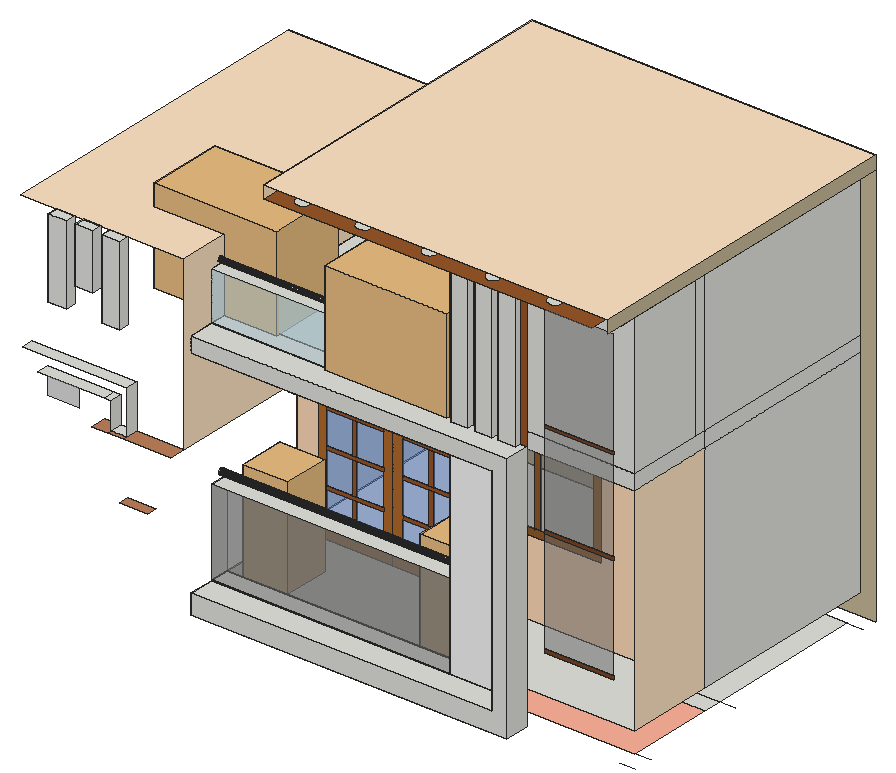
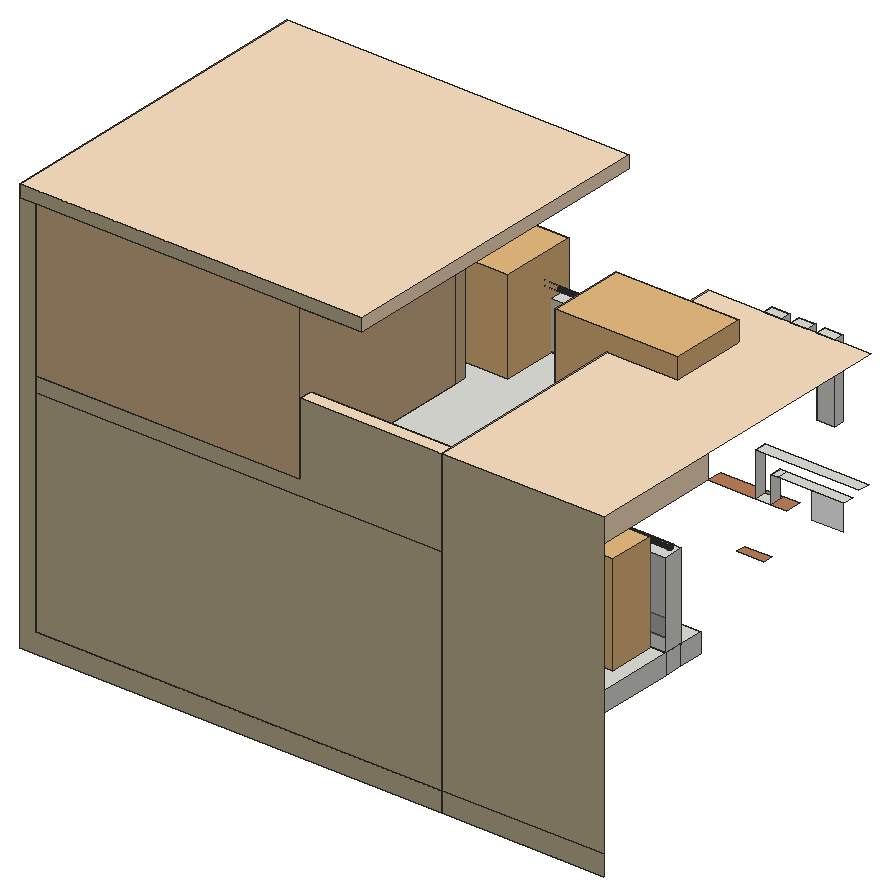
# SketchUp Ruby script. Lengths in inches.
U = 1.inch
M = Sketchup.active_model
def pt(a) = Geom::Point3d.new(a.map { |v| v * U })
def face(e, loops, mat)
  f = e.add_face(loops[0].map { |a| pt(a) })
  loops[1..].each { |l| e.add_face(l.map { |a| pt(a) }).erase! }
  f.material = f.back_material = mat if mat
  f
end
# faces: each face lists its corners as indices into pts; further lists are holes
def faces(e, pts, list, mat = nil) = list.each { |f| face(e, (f[0].is_a?(Array) ? f : [f]).map { |l| l.map { |i| pts[i] } }, mat) }
# xy, xz, yz: faces in a plane at the given z, y or x. An outline is a flat list of corners, or four numbers for a rectangle; further outlines are holes
def ring(l) = l.size == 4 ? [[l[0], l[1]], [l[2], l[1]], [l[2], l[3]], [l[0], l[3]]] : l.each_slice(2).to_a
def flat(e, list, mat, &to3) = list.each { |f| face(e, (f[0].is_a?(Array) ? f : [f]).map { |l| ring(l).map { |u, v| to3.(u, v) } }, mat) }
def xy(e, z, list, mat = nil) = flat(e, list, mat) { |x, y| [x, y, z] }
def xz(e, y, list, mat = nil) = flat(e, list, mat) { |x, z| [x, y, z] }
def yz(e, x, list, mat = nil) = flat(e, list, mat) { |y, z| [x, y, z] }
def lines(e, pts, list) = list.each { |a, b| e.add_line(pt(pts[a]), pt(pts[b])) }
# prism: a flat outline (further loops are holes) pulled along v
def prism(e, loops, v, mat = nil)
  f = face(e, loops, mat); d = Geom::Vector3d.new(v.map { |x| x * U })
  f.pushpull(f.normal.samedirection?(d) ? d.length : -d.length)
end
def box(e, o, s, mat = nil) = prism(e, [[o, [o[0] + s[0], o[1], o[2]], [o[0] + s[0], o[1] + s[1], o[2]], [o[0], o[1] + s[1], o[2]]]], [0, 0, s[2]], mat)
def at(x, y, z, deg = 0) = Geom::Transformation.translation(pt([x, y, z])) * Geom::Transformation.rotation(ORIGIN, Z_AXIS, deg.degrees)
def axes(o, x, y, z) = Geom::Transformation.new([*x, 0, *y, 0, *z, 0, *pt(o).to_a, 1])
def part(name) = M.definitions.add(name)
# library, detail: a bought-in or finely detailed component or shape, given as its bounding box
def library(name, o, s) = part(name).tap { |d| box(d.entities, o, s) }
def detail(e, o, s) = box(e.add_group.entities, o, s)
def put(e, d, t, mat = nil) = e.add_instance(d, t).tap { |i| i.material = mat if mat }
def group(e, t, mat = nil) = e.add_group.tap { |g| g.transformation = t; g.material = mat if mat }.entities
root = M.entities
M.materials.add("[0012_Bisque]").color = [255, 228, 196]
M.materials.add("[0027_PeachPuff]").color = [255, 218, 185]
M.materials.add("[0035_Tan]").color = [210, 180, 140]
M.materials.add("[Checker Plate]").color = [245, 245, 245]
M.materials.add("[Color B02]").color = [255, 178, 153]
M.materials.add("[Formica Laminate Dark]").color = [50, 53, 60]
M.materials.add("[Quartz Light Brown]1").color = [199, 184, 152]
M.materials.add("[Terrazzo Light Blue]").color = [196, 214, 227]
M.materials.add("[Terrazzo Tile Light]").color = [219, 217, 210]
M.materials.add("[Translucent Glass Blue]").color = [100, 149, 237]
M.materials["[Translucent Glass Blue]"].alpha = 0.5
M.materials.add("[Translucent Glass Gray]").color = [128, 128, 128]
M.materials["[Translucent Glass Gray]"].alpha = 0.5
M.materials.add("[Translucent Glass Safety]").color = [204, 235, 244]
M.materials["[Translucent Glass Safety]"].alpha = 0.5
M.materials.add("[Wood Bamboo]").color = [177, 105, 43]
M.materials.add("[Wood Cherry Original]").color = [152, 86, 42]
M.materials.add("[Wood Floor Parquet]").color = [145, 89, 39]
M.materials.add("[Wood Veneer 01]").color = [120, 70, 37]
M.materials.add("[Wood Veneer 02]").color = [190, 128, 91]
c1 = library("SPIKED_SUCCULENT_skp2020",[-8.43,-6.07,-0.04],[14.15,14.04,18.09])
c2 = library("Sem+nome",[-20.92,-6.25,0],[92.79,42.83,52.11])
xy(root,273.375,[[295.61,128.11,428.67,142.27],[428.67,128.11,471.875,142.27],[310.21,155.15,308.48,155.38,306.87,156.05,305.48,157.11,304.42,158.49,303.75,160.11,303.52,161.84,303.75,163.57,304.42,165.18,305.48,166.57,306.87,167.63,308.48,168.3,310.21,168.53,311.94,168.3,313.55,167.63,314.94,166.57,316,165.18,316.67,163.57,316.9,161.84,316.67,160.11,316,158.49,314.94,157.11,313.55,156.05,311.94,155.38],[358.27,155.15,356.54,155.38,354.93,156.05,353.54,157.11,352.48,158.49,351.8125,160.11,351.59,161.84,351.8125,163.57,352.48,165.18,353.54,166.57,354.93,167.63,356.54,168.3,358.27,168.53,360,168.3,361.62,167.63,363,166.57,364.06,165.18,364.73,163.57,364.96,161.84,364.73,160.11,364.06,158.49,363,157.11,361.62,156.05,360,155.38],[411.21,155.15,409.48,155.38,407.87,156.05,406.48,157.11,405.42,158.49,404.75,160.11,404.52,161.84,404.75,163.57,405.42,165.18,406.48,166.57,407.87,167.63,409.48,168.3,411.21,168.53,412.94,168.3,414.55,167.63,415.94,166.57,417,165.18,417.67,163.57,417.9,161.84,417.67,160.11,417,158.49,415.94,157.11,414.55,156.05,412.94,155.38],
  [295.61,201.9,523.42,212.08],[295.61,212.08,523.42,301.21],[227.05,301.21,295.61,310.21]])
xy(root,273.375,[[[295.61,142.27,295.61,201.9,523.42,201.9,523.42,152.96,428.67,152.96,428.67,142.27],[411.21,155.15,412.94,155.38,414.55,156.05,415.94,157.11,417,158.49,417.67,160.11,417.9,161.84,417.67,163.57,417,165.18,415.94,166.57,414.55,167.63,412.94,168.3,411.21,168.53,409.48,168.3,407.87,167.63,406.48,166.57,405.42,165.18,404.75,163.57,404.52,161.84,404.75,160.11,405.42,158.49,406.48,157.11,407.87,156.05,409.48,155.38],[358.27,155.15,360,155.38,361.62,156.05,363,157.11,364.06,158.49,364.73,160.11,364.96,161.84,364.73,163.57,364.06,165.18,363,166.57,361.62,167.63,360,168.3,358.27,168.53,356.54,168.3,354.93,167.63,353.54,166.57,352.48,165.18,351.8125,163.57,351.59,161.84,351.8125,160.11,352.48,158.49,353.54,157.11,354.93,156.05,356.54,155.38],[310.21,155.15,311.94,155.38,313.55,156.05,314.94,157.11,316,158.49,316.67,160.11,316.9,161.84,316.67,163.57,316,165.18,314.94,166.57,313.55,167.63,311.94,168.3,310.21,168.53,308.48,168.3,306.87,167.63,305.48,166.57,304.42,165.18,303.75,163.57,303.52,161.84,303.75,160.11,304.42,158.49,305.48,157.11,306.87,156.05,308.48,155.38]]],"[Color B02]")
xy(root,284.5625,[[295.61,128.11,463.72,142.27],[295.61,142.27,428.67,152.96],[295.61,152.96,523.42,201.9],[295.61,201.9,523.42,310.21]])
xy(root,284.6875,[[295.61,142.27,428.67,152.96]])
xy(root,325.82,[[267.29,113.95,282.48,119.57]],"[Wood Veneer 02]")
xy(root,332.6875,[[295.61,142.27,428.67,152.96]])
xy(root,358.46,[[260.41,116.39,269.14,122.95]])
xy(root,358.46,[[251.36,113.95,260.41,122.95],[260.41,113.95,269.14,116.39],[269.14,113.95,295.61,122.95]],"[Wood Veneer 02]")
xy(root,373.65,[[219.57,116.39,256.72,122.95],[256.72,116.39,260.41,122.95]])
xy(root,383.14,[[210.89,116.39,269.14,122.95]])
xy(root,404.5625,[[295.61,128.11,428.67,142.27],[428.67,128.11,463.72,142.27],[308.49,153.67,306.91,153.875,305.43,154.49,304.16,155.46,303.19,156.73,302.58,158.21,302.37,159.79,302.58,161.38,303.19,162.85,304.16,164.12,305.43,165.1,306.91,165.71,308.49,165.92,310.08,165.71,311.56,165.1,312.83,164.12,313.8,162.85,314.41,161.38,314.62,159.79,314.41,158.21,313.8,156.73,312.83,155.46,311.56,154.49,310.08,153.875],[359.37,153.67,357.78,153.875,356.31,154.49,355.04,155.46,354.06,156.73,353.45,158.21,353.24,159.79,353.45,161.38,354.06,162.85,355.04,164.12,356.31,165.1,357.78,165.71,359.37,165.92,360.95,165.71,362.43,165.1,363.7,164.12,364.67,162.85,365.29,161.38,365.49,159.79,365.29,158.21,364.67,156.73,363.7,155.46,362.43,154.49,360.95,153.875],[409.62,153.67,408.03,153.875,406.56,154.49,405.29,155.46,404.31,156.73,403.7,158.21,403.49,159.79,403.7,161.38,404.31,162.85,405.29,164.12,406.56,165.1,408.03,165.71,409.62,165.92,411.2,165.71,412.68,165.1,413.95,164.12,414.92,162.85,415.54,161.38,415.74,159.79,415.54,158.21,414.92,156.73,413.95,155.46,412.68,154.49,411.2,153.875],
  [295.61,201.9,375.08,302.74],[375.08,201.9,375.08,302.74,295.61,302.74,295.61,310.21,523.42,310.21,523.42,201.9]])
xy(root,404.5625,[[[295.61,142.27,295.61,201.9,523.42,201.9,523.42,152.96,428.67,153.15,428.67,142.27],[409.62,153.67,411.2,153.875,412.68,154.49,413.95,155.46,414.92,156.73,415.54,158.21,415.74,159.79,415.54,161.38,414.92,162.85,413.95,164.12,412.68,165.1,411.2,165.71,409.62,165.92,408.03,165.71,406.56,165.1,405.29,164.12,404.31,162.85,403.7,161.38,403.49,159.79,403.7,158.21,404.31,156.73,405.29,155.46,406.56,154.49,408.03,153.875],[359.37,153.67,360.95,153.875,362.43,154.49,363.7,155.46,364.67,156.73,365.29,158.21,365.49,159.79,365.29,161.38,364.67,162.85,363.7,164.12,362.43,165.1,360.95,165.71,359.37,165.92,357.78,165.71,356.31,165.1,355.04,164.12,354.06,162.85,353.45,161.38,353.24,159.79,353.45,158.21,354.06,156.73,355.04,155.46,356.31,154.49,357.78,153.875],[308.49,153.67,310.08,153.875,311.56,154.49,312.83,155.46,313.8,156.73,314.41,158.21,314.62,159.79,314.41,161.38,313.8,162.85,312.83,164.12,311.56,165.1,310.08,165.71,308.49,165.92,306.91,165.71,305.43,165.1,304.16,164.12,303.19,162.85,302.58,161.38,302.37,159.79,302.58,158.21,303.19,156.73,304.16,155.46,305.43,154.49,306.91,153.875]]],"[Color B02]")
xy(root,410.0625,[[224.59,117.2,234.84,122.95],[254.28,117.2,264.53,122.95]])
xy(root,413.375,[[295.61,128.11,471.875,128.11,471.875,142.27,467.89,142.27,467.89,139.08,458.27,139.08,458.27,142.27,454.71,142.27,454.71,139.08,445.08,139.08,445.08,142.27,441.39,142.27,441.39,139.08,431.77,139.08,431.77,142.27,295.61,142.27],[431.77,139.08,441.39,142.27],[445.08,139.08,454.71,142.27],[458.27,139.08,467.89,142.27],[295.61,142.27,428.67,142.27,428.67,153.15,295.61,152.96],
  [295.61,152.96,428.67,153.15,523.42,152.96,523.42,194.54,375.08,194.54,375.08,302.74,295.61,302.74],[375.08,194.54,523.42,201.9],[375.08,201.9,523.42,310.21]])
xy(root,423.25,[[239.66,117.2,249.35,122.95]])
xy(root,440.625,[[295.61,142.27,428.67,142.27,428.67,153.15,295.61,152.96]])
xy(root,454.0625,[[224.59,117.2,234.84,122.95],[239.66,117.2,249.35,122.95],[254.28,117.2,264.53,122.95]])
xy(root,454.0625,[[204.37,122.95,295.61,310.21],[295.61,302.74,375.08,310.21]],"[0012_Bisque]")
xy(root,494.4375,[[431.77,139.08,441.39,142.27],[445.08,139.08,454.71,142.27],[458.27,139.08,467.89,142.27]])
xy(root,499.5,[[355.18,128.13,354.18,128.26,353.24,128.65,352.44,129.27,351.83,130.07,351.4375,131,351.31,132.01,351.4375,133.01,351.83,133.94,352.44,134.75,353.24,135.36,354.18,135.75,355.18,135.88,356.19,135.75,357.12,135.36,357.92,134.75,358.54,133.94,358.93,133.01,359.06,132.01,358.93,131,358.54,130.07,357.92,129.27,357.12,128.65,356.19,128.26],[389.06,128.13,388.05,128.26,387.12,128.65,386.32,129.27,385.7,130.07,385.3125,131,385.18,132.01,385.3125,133.01,385.7,133.94,386.32,134.75,387.12,135.36,388.05,135.75,389.06,135.88,390.06,135.75,390.99,135.36,391.8,134.75,392.41,133.94,392.8,133.01,392.93,132.01,392.8,131,392.41,130.07,391.8,129.27,390.99,128.65,390.06,128.26],[425.93,128.13,424.93,128.26,423.99,128.65,423.19,129.27,422.58,130.07,422.1875,131,422.06,132.01,422.1875,133.01,422.58,133.94,423.19,134.75,423.99,135.36,424.93,135.75,425.93,135.88,426.94,135.75,427.87,135.36,428.67,134.75,429.29,133.94,429.68,133.01,429.81,132.01,429.68,131,429.29,130.07,428.67,129.27,427.87,128.65,426.94,128.26],[461.12,128.13,460.12,128.26,459.18,128.65,458.38,129.27,457.76,130.07,457.375,131,457.24,132.01,457.375,133.01,457.76,133.94,458.38,134.75,459.18,135.36,460.12,135.75,461.12,135.88,462.12,135.75,463.06,135.36,463.86,134.75,464.48,133.94,464.86,133.01,464.99,132.01,464.86,131,464.48,130.07,463.86,129.27,463.06,128.65,462.12,128.26],[495.93,128.13,494.93,128.26,493.99,128.65,493.19,129.27,492.58,130.07,492.1875,131,492.06,132.01,492.1875,133.01,492.58,133.94,493.19,134.75,493.99,135.36,494.93,135.75,495.93,135.88,496.94,135.75,497.87,135.36,498.67,134.75,499.29,133.94,499.68,133.01,499.81,132.01,499.68,131,499.29,130.07,498.67,129.27,497.87,128.65,496.94,128.26],
  [523.42,132.61,532.42,142.27],[428.67,142.27,428.67,153.15,523.42,152.96,532.42,152.96,532.42,142.27],[523.42,152.96,532.42,194.54],[375.08,194.54,523.42,201.9],[523.42,194.54,532.42,201.9],
  [375.08,201.9,523.42,310.21],[523.42,201.9,532.42,310.21]])
xy(root,499.5,[[[340.2,122.95,340.2,310.21,375.08,310.21,375.08,194.54,523.42,194.54,523.42,152.96,428.67,153.15,428.67,142.27,523.42,142.27,523.42,122.95],[355.18,128.13,356.19,128.26,357.12,128.65,357.92,129.27,358.54,130.07,358.93,131,359.06,132.01,358.93,133.01,358.54,133.94,357.92,134.75,357.12,135.36,356.19,135.75,355.18,135.88,354.18,135.75,353.24,135.36,352.44,134.75,351.83,133.94,351.4375,133.01,351.31,132.01,351.4375,131,351.83,130.07,352.44,129.27,353.24,128.65,354.18,128.26],[461.12,128.13,462.12,128.26,463.06,128.65,463.86,129.27,464.48,130.07,464.86,131,464.99,132.01,464.86,133.01,464.48,133.94,463.86,134.75,463.06,135.36,462.12,135.75,461.12,135.88,460.12,135.75,459.18,135.36,458.38,134.75,457.76,133.94,457.375,133.01,457.24,132.01,457.375,131,457.76,130.07,458.38,129.27,459.18,128.65,460.12,128.26],[389.06,128.13,390.06,128.26,390.99,128.65,391.8,129.27,392.41,130.07,392.8,131,392.93,132.01,392.8,133.01,392.41,133.94,391.8,134.75,390.99,135.36,390.06,135.75,389.06,135.88,388.05,135.75,387.12,135.36,386.32,134.75,385.7,133.94,385.3125,133.01,385.18,132.01,385.3125,131,385.7,130.07,386.32,129.27,387.12,128.65,388.05,128.26],[495.93,128.13,496.94,128.26,497.87,128.65,498.67,129.27,499.29,130.07,499.68,131,499.81,132.01,499.68,133.01,499.29,133.94,498.67,134.75,497.87,135.36,496.94,135.75,495.93,135.88,494.93,135.75,493.99,135.36,493.19,134.75,492.58,133.94,492.1875,133.01,492.06,132.01,492.1875,131,492.58,130.07,493.19,129.27,493.99,128.65,494.93,128.26],[425.93,128.13,426.94,128.26,427.87,128.65,428.67,129.27,429.29,130.07,429.68,131,429.81,132.01,429.68,133.01,429.29,133.94,428.67,134.75,427.87,135.36,426.94,135.75,425.93,135.88,424.93,135.75,423.99,135.36,423.19,134.75,422.58,133.94,422.1875,133.01,422.06,132.01,422.1875,131,422.58,130.07,423.19,129.27,423.99,128.65,424.93,128.26]]],"[Wood Cherry Original]")
xy(root,506.6875,[[340.2,122.95,532.42,310.21]],"[0012_Bisque]")
xz(root,117.2,[[224.59,410.0625,234.84,454.0625],[254.28,410.0625,264.53,454.0625],[239.66,423.25,249.35,454.0625]])
xz(root,122.95,[[224.59,410.0625,234.84,454.0625],[254.28,410.0625,264.53,454.0625],[239.66,423.25,249.35,454.0625]])
xz(root,122.95,[[219.6,358.46,237.54,358.46,237.54,373.65,219.57,373.65]],"[Translucent Glass Gray]")
xz(root,128.11,[[295.61,273.375,471.875,273.375,471.875,413.375,295.61,413.375,295.61,404.5625,463.72,404.5625,463.72,284.5625,295.61,284.5625]])
xz(root,139.08,[[431.77,413.375,441.39,494.4375],[445.08,413.375,454.71,494.4375],[458.27,413.375,467.89,494.4375]])
xz(root,142.27,[[295.61,273.375,295.61,284.5625,463.72,284.5625,463.72,404.5625,471.875,404.5625,471.875,273.375],[295.61,284.5625,428.67,284.6875],[295.61,404.5625,428.67,413.375],[428.67,404.5625,471.875,413.375],[431.77,413.375,441.39,494.4375],
  [445.08,413.375,454.71,494.4375],[458.27,413.375,467.89,494.4375]])
xz(root,142.27,[[428.67,284.5625,463.72,404.5625]],"[Checker Plate]")
xz(root,142.27,[[295.61,284.6875,428.67,332.6875],[481.64,315.75,520.01,373.43],[481.64,375.31,520.01,426.06],[481.64,427.93,520.01,486.71]],"[Translucent Glass Gray]")
xz(root,142.27,[[295.61,413.375,428.67,440.625]],"[Translucent Glass Safety]")
xz(root,142.27,[[428.67,413.375,431.77,413.375,431.77,494.4375,441.39,494.4375,441.39,413.375,445.08,413.375,445.08,494.4375,454.71,494.4375,454.71,413.375,458.27,413.375,458.27,494.4375,467.89,494.4375,467.89,413.375,471.875,413.375,471.875,499.5,428.67,499.5]],"[Wood Cherry Original]")
xz(root,142.27,[[481.64,313.87,520.01,315.75],[481.64,373.43,520.01,375.31],[481.64,426.06,520.01,427.93]],"[Wood Veneer 01]")
xz(root,152.96,[[295.61,284.5625,428.67,284.6875]])
xz(root,152.96,[[295.61,284.6875,428.67,332.6875]],"[Translucent Glass Gray]")
xz(root,194.54,[[[375.08,413.375,523.42,499.5],[383.18,435.35,413.43,484.29],[429.81,435.35,460.06,484.29]]],"[0035_Tan]")
xz(root,194.54,[[386.91,439.08,409.7,480.5625],[433.53,439.08,456.33,480.5625]],"[Translucent Glass Gray]")
xz(root,194.54,[[[383.18,435.35,413.43,484.29],[386.91,439.08,409.7,480.5625]],[[429.81,435.35,460.06,484.29],[433.53,439.08,456.33,480.5625]]],"[Wood Veneer 01]")
xz(root,201.9,[[375.08,404.5625,523.42,413.375],[375.08,413.375,523.42,499.5]])
xz(root,201.9,[[[295.61,284.5625,307.11,284.5625,307.11,393.3125,391.68,393.3125,391.68,284.5625,523.42,284.5625,523.42,404.5625,295.61,404.5625],[398.3,326.375,465.61,393.6875],[297.54,378.85,304.1,394.62]]],"[0027_PeachPuff]")
xz(root,201.9,[[297.54,378.85,304.1,394.62]],"[Formica Laminate Dark]")
xz(root,201.9,[[312.21,289.66,326.86,309.625],[329.17,289.66,344.3,309.625],[354.49,289.66,369.24,309.625],[371.89,289.66,386.58,309.625],[312.21,311.61,326.86,329.59],
  [329.17,311.61,344.3,329.59],[354.49,311.61,369.24,329.59],[371.89,311.61,386.58,329.59],[312.21,331.58,326.86,349.72],[329.17,331.58,344.3,349.72],
  [354.49,331.58,369.24,349.72],[371.89,331.58,386.58,349.72],[312.21,351.7,326.86,368.34],[329.17,351.7,344.3,368.34],[354.49,351.7,369.24,368.34],
  [371.89,351.7,386.58,368.34],[312.21,370.33,326.86,388.22],[329.17,370.33,344.3,388.22],[354.49,370.33,369.24,388.22],[371.89,370.33,386.58,388.22]],"[Translucent Glass Blue]")
xz(root,201.9,[[402.61,330.69,428.67,389.37],[432.04,330.69,461.3,389.37]],"[Translucent Glass Gray]")
xz(root,201.9,[[[307.11,284.5625,349.4,393.3125],[312.21,289.66,344.3,388.22]],[[349.4,284.5625,391.68,393.3125],[354.49,289.66,386.58,388.22]]],"[Wood Bamboo]")
xz(root,201.9,[[326.86,289.66,329.17,309.625],[369.24,289.66,371.89,309.625],[312.21,309.625,344.3,311.61],[354.49,309.625,386.58,311.61],[326.86,311.61,329.17,329.59],
  [369.24,311.61,371.89,329.59],[312.21,329.59,344.3,331.58],[354.49,329.59,386.58,331.58],[326.86,331.58,329.17,349.72],[369.24,331.58,371.89,349.72],
  [312.21,349.72,344.3,351.7],[354.49,349.72,386.58,351.7],[326.86,351.7,329.17,368.34],[369.24,351.7,371.89,368.34],[312.21,368.34,344.3,370.33],
  [354.49,368.34,386.58,370.33],[326.86,370.33,329.17,388.22],[369.24,370.33,371.89,388.22]],"[Wood Cherry Original]")
xz(root,201.9,[[[398.3,326.375,465.61,393.6875],[402.61,330.69,461.3,389.37]],[428.67,330.69,432.04,389.37]],"[Wood Floor Parquet]")
xz(root,302.74,[[295.61,404.5625,375.08,413.375]])
xz(root,302.74,[[295.61,413.375,375.08,454.0625]],"[0012_Bisque]")
xz(root,310.21,[[375.08,413.375,523.42,499.5]],"[0035_Tan]")
xz(root,310.21,[[204.37,273.375,295.61,284.5625],[295.61,273.375,295.61,284.5625,523.42,284.5625,523.42,499.5,532.42,499.5,532.42,273.375],[204.37,284.5625,295.61,454.0625],[295.61,284.5625,523.42,404.5625],[295.61,404.5625,295.61,454.0625,375.08,454.0625,375.08,413.375,523.42,413.375,523.42,404.5625],
  [340.2,499.5,532.42,506.6875]],"[Quartz Light Brown]1")
yz(root,224.59,[[117.2,410.0625,122.95,454.0625]])
yz(root,234.84,[[117.2,410.0625,122.95,454.0625]])
yz(root,239.66,[[117.2,423.25,122.95,454.0625]])
yz(root,249.35,[[117.2,423.25,122.95,454.0625]])
yz(root,254.28,[[117.2,410.0625,122.95,454.0625]])
yz(root,260.41,[[116.39,358.46,122.95,373.65]])
yz(root,264.53,[[117.2,410.0625,122.95,454.0625]])
yz(root,269.14,[[116.39,358.46,122.95,383.14]])
yz(root,295.61,[[128.11,273.375,142.27,284.5625],[142.27,273.375,152.96,284.5625],[152.96,273.375,201.9,284.5625],[201.9,273.375,212.08,284.5625],[212.08,273.375,310.21,284.5625],
  [142.27,284.5625,152.96,284.6875],[201.9,284.5625,310.21,404.5625],[142.27,284.6875,152.96,332.6875],[128.11,404.5625,132.61,413.375],[132.61,404.5625,142.27,413.375],
  [142.27,404.5625,152.96,413.375],[152.96,404.5625,201.9,413.375],[201.9,404.5625,302.74,413.375],[302.74,404.5625,310.21,454.0625],[142.27,413.375,152.96,440.625]])
yz(root,295.61,[[[122.95,358.46,201.9,358.46,201.9,404.5625,128.11,404.5625,128.11,413.375,142.27,413.375,142.27,440.625,152.96,440.625,152.96,413.375,302.74,413.375,302.74,454.0625,122.95,454.0625],[147.66,441.9,147.36,441.9375,147.07,442.06,146.82,442.24,146.64,442.49,146.52,442.78,146.48,443.08,146.52,443.39,146.64,443.68,146.82,443.92,147.07,444.11,147.36,444.23,147.66,444.27,147.97,444.23,148.26,444.11,148.5,443.92,148.69,443.68,148.81,443.39,148.85,443.08,148.81,442.78,148.69,442.49,148.5,442.24,148.26,442.06,147.97,441.9375]]],"[0012_Bisque]")
yz(root,340.2,[[122.95,499.5,310.21,506.6875]],"[0012_Bisque]")
yz(root,375.08,[[201.9,404.5625,302.74,413.375],[302.74,413.375,310.21,454.0625]])
yz(root,375.08,[[194.54,413.375,201.9,499.5],[201.9,413.375,201.9,499.5,310.21,499.5,310.21,454.0625,302.74,454.0625,302.74,413.375]],"[0035_Tan]")
yz(root,428.67,[[142.27,284.5625,152.96,284.6875],[142.27,284.6875,152.96,332.6875],[148.83,334.82,149.22,334.87,149.58,335.02,149.89,335.26,150.13,335.57,150.28,335.93,150.33,336.32,150.28,336.7,150.13,337.07,149.89,337.38,149.58,337.62,149.22,337.77,148.83,337.82,148.44,337.77,148.08,337.62,147.77,337.38,147.53,337.07,147.38,336.7,147.33,336.32,147.38,335.93,147.53,335.57,147.77,335.26,148.08,335.02,148.44,334.87],[142.27,404.5625,153.15,413.375],[142.27,413.375,153.15,440.625],
  [[142.27,440.625,153.15,499.5],[147.66,441.9,147.97,441.9375,148.26,442.06,148.5,442.24,148.69,442.49,148.81,442.78,148.85,443.08,148.81,443.39,148.69,443.68,148.5,443.92,148.26,444.11,147.97,444.23,147.66,444.27,147.36,444.23,147.07,444.11,146.82,443.92,146.64,443.68,146.52,443.39,146.48,443.08,146.52,442.78,146.64,442.49,146.82,442.24,147.07,442.06,147.36,441.9375]],[147.66,441.9,147.97,441.9375,148.26,442.06,148.5,442.24,148.69,442.49,148.81,442.78,148.85,443.08,148.81,443.39,148.69,443.68,148.5,443.92,148.26,444.11,147.97,444.23,147.66,444.27,147.36,444.23,147.07,444.11,146.82,443.92,146.64,443.68,146.52,443.39,146.48,443.08,146.52,442.78,146.64,442.49,146.82,442.24,147.07,442.06,147.36,441.9375]])
yz(root,428.67,[[[142.27,332.6875,152.96,404.5625],[148.83,334.82,149.22,334.87,149.58,335.02,149.89,335.26,150.13,335.57,150.28,335.93,150.33,336.32,150.28,336.7,150.13,337.07,149.89,337.38,149.58,337.62,149.22,337.77,148.83,337.82,148.44,337.77,148.08,337.62,147.77,337.38,147.53,337.07,147.38,336.7,147.33,336.32,147.38,335.93,147.53,335.57,147.77,335.26,148.08,335.02,148.44,334.87]]],"[0027_PeachPuff]")
yz(root,431.77,[[139.08,413.375,142.27,494.4375]])
yz(root,441.39,[[139.08,413.375,142.27,494.4375]])
yz(root,445.08,[[139.08,413.375,142.27,494.4375]])
yz(root,454.71,[[139.08,413.375,142.27,494.4375]])
yz(root,458.27,[[139.08,413.375,142.27,494.4375]])
yz(root,463.72,[[128.11,284.5625,142.27,404.5625]])
yz(root,467.89,[[139.08,413.375,142.27,494.4375]])
yz(root,471.875,[[128.11,273.375,142.27,413.375]])
yz(root,523.42,[[201.9,284.5625,310.21,404.5625],[152.96,404.5625,201.9,413.375],[201.9,404.5625,310.21,413.375],[152.96,413.375,194.54,499.5],[194.54,413.375,201.9,499.5],
  [201.9,413.375,310.21,499.5]])
yz(root,523.42,[[152.96,284.5625,201.9,404.5625]],"[0012_Bisque]")
yz(root,532.42,[[122.95,499.5,310.21,506.6875]],"[Quartz Light Brown]1")
p = [[428.67,148.83,334.82],[428.67,148.44,334.87],[295.61,148.44,334.87],[295.61,148.83,334.82],[428.67,149.22,334.87],[295.61,149.22,334.87],
  [428.67,148.08,335.02],[295.61,148.08,335.02],[428.67,149.58,335.02],[295.61,149.58,335.02],[428.67,147.77,335.26],[295.61,147.77,335.26],
  [428.67,149.89,335.26],[295.61,149.89,335.26],[428.67,147.53,335.57],[295.61,147.53,335.57],[428.67,150.13,335.57],[295.61,150.13,335.57],
  [428.67,147.38,335.93],[295.61,147.38,335.93],[428.67,150.28,335.93],[295.61,150.28,335.93],[428.67,147.33,336.32],[295.61,147.33,336.32],
  [428.67,150.33,336.32],[295.61,150.33,336.32],[428.67,147.38,336.7],[295.61,147.38,336.7],[428.67,150.28,336.7],[295.61,150.28,336.7],
  [428.67,147.53,337.07],[295.61,147.53,337.07],[428.67,150.13,337.07],[295.61,150.13,337.07],[428.67,147.77,337.38],[295.61,147.77,337.38],
  [428.67,149.89,337.38],[295.61,149.89,337.38],[428.67,148.08,337.62],[295.61,148.08,337.62],[428.67,149.58,337.62],[295.61,149.58,337.62],
  [428.67,148.44,337.77],[295.61,148.44,337.77],[428.67,149.22,337.77],[295.61,149.22,337.77],[428.67,148.83,337.82],[295.61,148.83,337.82],
  [523.42,152.96,413.375],[428.67,153.15,413.375],[428.67,153.15,404.5625],[523.42,152.96,404.5625],[295.61,152.96,413.375],[295.61,152.96,440.625],
  [428.67,153.15,440.625],[428.67,153.15,499.5],[523.42,152.96,499.5],[428.67,147.36,441.9375],[428.67,147.07,442.06],[295.61,147.07,442.06],
  [295.61,147.36,441.9375],[428.67,147.66,441.9],[295.61,147.66,441.9],[428.67,147.97,441.9375],[295.61,147.97,441.9375],[428.67,148.26,442.06],
  [295.61,148.26,442.06],[428.67,146.82,442.24],[295.61,146.82,442.24],[428.67,148.5,442.24],[295.61,148.5,442.24],[428.67,146.64,442.49],
  [295.61,146.64,442.49],[428.67,148.69,442.49],[295.61,148.69,442.49],[428.67,146.52,442.78],[295.61,146.52,442.78],[428.67,148.81,442.78],
  [295.61,148.81,442.78],[428.67,146.48,443.08],[295.61,146.48,443.08],[428.67,148.85,443.08],[295.61,148.85,443.08],[428.67,146.52,443.39],
  [295.61,146.52,443.39],[428.67,148.81,443.39],[295.61,148.81,443.39],[428.67,146.64,443.68],[295.61,146.64,443.68],[428.67,148.69,443.68],
  [295.61,148.69,443.68],[428.67,146.82,443.92],[295.61,146.82,443.92],[428.67,148.5,443.92],[295.61,148.5,443.92],[428.67,147.07,444.11],
  [295.61,147.07,444.11],[428.67,148.26,444.11],[295.61,148.26,444.11],[428.67,147.36,444.23],[295.61,147.36,444.23],[428.67,147.97,444.23],
  [295.61,147.97,444.23],[428.67,147.66,444.27],[295.61,147.66,444.27],[523.42,301.21,273.375],[532.42,301.21,273.375],[523.42,212.08,273.375],
  [532.42,212.08,273.375],[523.42,142.27,273.375],[532.42,142.27,273.375],[523.42,152.96,273.375],[532.42,152.96,273.375]]
faces(root,p,[[0,1,2,3],[4,0,3,5],[1,6,7,2],[8,4,5,9],[6,10,11,7],[12,8,9,13],[10,14,15,11],[16,12,13,17],
  [14,18,19,15],[20,16,17,21],[18,22,23,19],[24,20,21,25],[22,26,27,23],[28,24,25,29],[26,30,31,27],[32,28,29,33],
  [30,34,35,31],[36,32,33,37],[34,38,39,35],[40,36,37,41],[38,42,43,39],[44,40,41,45],[42,46,47,43],[46,44,45,47]],"[Terrazzo Light Blue]")
faces(root,p,[[48,49,50,51],[48,49,54,55,56]])
faces(root,p,[[49,52,53,54]],"[Translucent Glass Safety]")
faces(root,p,[[57,58,59,60],[61,57,60,62],[63,61,62,64],[65,63,64,66],[58,67,68,59],[69,65,66,70],[67,71,72,68],[73,69,70,74],
  [71,75,76,72],[77,73,74,78],[75,79,80,76],[81,77,78,82],[79,83,84,80],[85,81,82,86],[83,87,88,84],[89,85,86,90],
  [87,91,92,88],[93,89,90,94],[91,95,96,92],[97,93,94,98],[95,99,100,96],[101,97,98,102],[99,103,104,100],[103,101,102,104]],"[Terrazzo Tile Light]")
lines(root,p,[[105,106],[107,108],[109,110],[111,112]])
put(root,c1,axes([318.92,164.73,284.69],[1.78,0,0],[0,1.85,0],[0,0,3.09617]))
put(root,c1,axes([418.23,164.73,284.69],[1.78,0,0],[0,1.85,0],[0,0,3.09617]))
put(root,c2,axes([271.67,157.32,413.375],[0.7392,0,0],[0,1,0],[0,0,1]))
put(root,c2,axes([375.54,146.77,413.375],[0.7392,0,0],[0,1,0],[0,0,1]))
